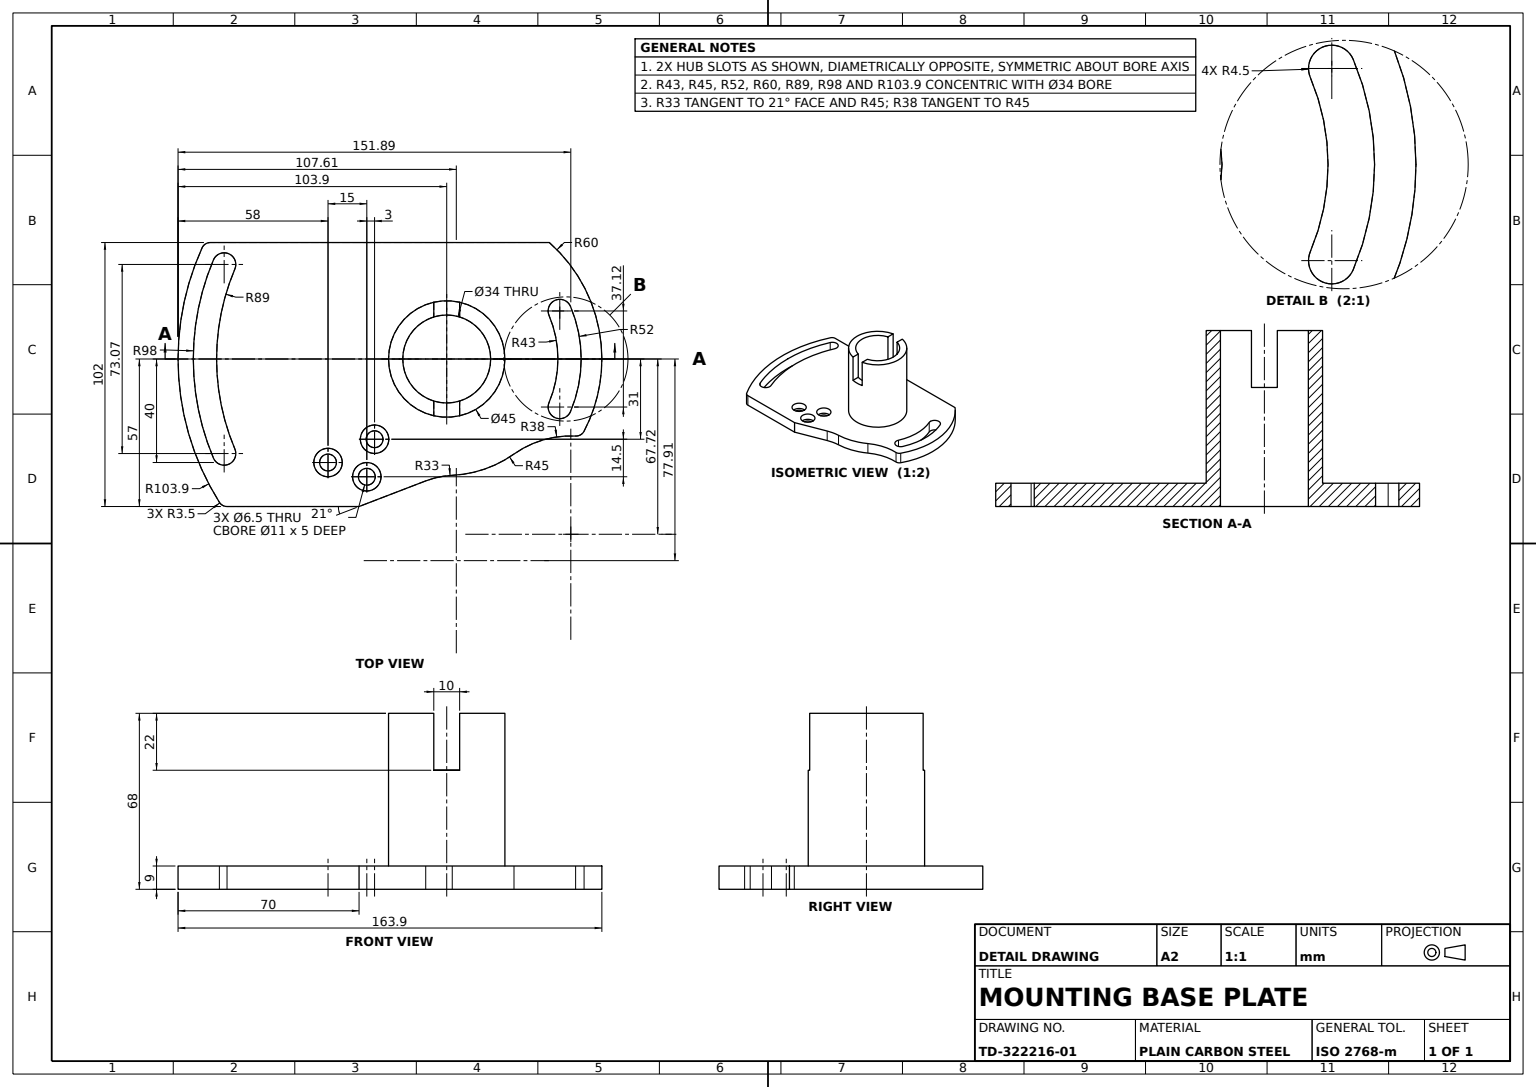
ISO-10303-21;
HEADER;
FILE_DESCRIPTION((''),'2;1');
FILE_NAME('','',(''),(''),'','','');
FILE_SCHEMA(('AUTOMOTIVE_DESIGN'));
ENDSEC;
DATA;
#1=APPLICATION_CONTEXT('');
#2=PRODUCT_CONTEXT('',#1,'mechanical');
#3=PRODUCT('','','',(#2));
#4=PRODUCT_DEFINITION_FORMATION('','',#3);
#5=PRODUCT_DEFINITION_CONTEXT('',#1,'design');
#6=PRODUCT_DEFINITION('','',#4,#5);
#7=PRODUCT_DEFINITION_SHAPE('','',#6);
#8=(LENGTH_UNIT()NAMED_UNIT(*)SI_UNIT(.MILLI.,.METRE.));
#9=(NAMED_UNIT(*)PLANE_ANGLE_UNIT()SI_UNIT($,.RADIAN.));
#10=(NAMED_UNIT(*)SI_UNIT($,.STERADIAN.)SOLID_ANGLE_UNIT());
#11=UNCERTAINTY_MEASURE_WITH_UNIT(LENGTH_MEASURE(1.E-05),#8,'distance_accuracy_value','');
#12=(GEOMETRIC_REPRESENTATION_CONTEXT(3)GLOBAL_UNCERTAINTY_ASSIGNED_CONTEXT((#11))GLOBAL_UNIT_ASSIGNED_CONTEXT((#8,#9,#10))REPRESENTATION_CONTEXT('',''));
#13=CARTESIAN_POINT('',(55.36504,0.,87.919977));
#14=VERTEX_POINT('',#13);
#15=CARTESIAN_POINT('',(57.,0.,84.958284));
#16=VERTEX_POINT('',#15);
#17=CARTESIAN_POINT('',(53.5,0.,84.958284));
#18=DIRECTION('',(0.,1.,0.));
#19=DIRECTION('',(0.,0.,-1.));
#20=AXIS2_PLACEMENT_3D('',#17,#18,#19);
#21=CIRCLE('',#20,3.5);
#22=EDGE_CURVE('',#14,#16,#21,.T.);
#23=ORIENTED_EDGE('',*,*,#22,.T.);
#24=CARTESIAN_POINT('',(57.,9.,84.958284));
#25=VERTEX_POINT('',#24);
#26=DIRECTION('',(0.,-1.,0.));
#27=VECTOR('',#26,1000.);
#28=LINE('',#24,#27);
#29=EDGE_CURVE('',#25,#16,#28,.T.);
#30=ORIENTED_EDGE('',*,*,#29,.F.);
#31=CARTESIAN_POINT('',(55.36504,9.,87.919977));
#32=VERTEX_POINT('',#31);
#33=CARTESIAN_POINT('',(53.5,9.,84.958284));
#34=AXIS2_PLACEMENT_3D('',#33,#18,#19);
#35=CIRCLE('',#34,3.5);
#36=EDGE_CURVE('',#32,#25,#35,.T.);
#37=ORIENTED_EDGE('',*,*,#36,.F.);
#38=LINE('',#31,#27);
#39=EDGE_CURVE('',#32,#14,#38,.T.);
#40=ORIENTED_EDGE('',*,*,#39,.T.);
#41=EDGE_LOOP('',(#23,#30,#37,#40));
#42=FACE_OUTER_BOUND('',#41,.T.);
#43=AXIS2_PLACEMENT_3D('',#33,#26,#19);
#44=CYLINDRICAL_SURFACE('',#43,3.5);
#45=ADVANCED_FACE('',(#42),#44,.T.);
#46=CARTESIAN_POINT('',(40.,4.,40.4));
#47=VERTEX_POINT('',#46);
#48=CARTESIAN_POINT('',(40.,4.,51.4));
#49=VERTEX_POINT('',#48);
#50=CARTESIAN_POINT('',(40.,4.,45.9));
#51=DIRECTION('',(0.,0.,1.));
#52=AXIS2_PLACEMENT_3D('',#50,#18,#51);
#53=CIRCLE('',#52,5.5);
#54=EDGE_CURVE('',#47,#49,#53,.T.);
#55=ORIENTED_EDGE('',*,*,#54,.F.);
#56=CARTESIAN_POINT('',(40.,9.,40.4));
#57=VERTEX_POINT('',#56);
#58=VECTOR('',#18,1000.);
#59=LINE('',#56,#58);
#60=EDGE_CURVE('',#47,#57,#59,.T.);
#61=ORIENTED_EDGE('',*,*,#60,.T.);
#62=CARTESIAN_POINT('',(40.,9.,51.4));
#63=VERTEX_POINT('',#62);
#64=CARTESIAN_POINT('',(40.,9.,45.9));
#65=AXIS2_PLACEMENT_3D('',#64,#18,#51);
#66=CIRCLE('',#65,5.5);
#67=EDGE_CURVE('',#57,#63,#66,.T.);
#68=ORIENTED_EDGE('',*,*,#67,.T.);
#69=LINE('',#62,#58);
#70=EDGE_CURVE('',#49,#63,#69,.T.);
#71=ORIENTED_EDGE('',*,*,#70,.F.);
#72=EDGE_LOOP('',(#55,#61,#68,#71));
#73=FACE_OUTER_BOUND('',#72,.T.);
#74=CYLINDRICAL_SURFACE('',#65,5.5);
#75=ADVANCED_FACE('',(#73),#74,.F.);
#76=CARTESIAN_POINT('',(21.937411,68.,-5.));
#77=VERTEX_POINT('',#76);
#78=CARTESIAN_POINT('',(0.,68.,-22.5));
#79=VERTEX_POINT('',#78);
#80=CARTESIAN_POINT('',(0.,68.,0.));
#81=AXIS2_PLACEMENT_3D('',#80,#18,#51);
#82=CIRCLE('',#81,22.5);
#83=EDGE_CURVE('',#77,#79,#82,.T.);
#84=ORIENTED_EDGE('',*,*,#83,.T.);
#85=CARTESIAN_POINT('',(-21.937411,68.,-5.));
#86=VERTEX_POINT('',#85);
#87=EDGE_CURVE('',#79,#86,#82,.T.);
#88=ORIENTED_EDGE('',*,*,#87,.T.);
#89=CARTESIAN_POINT('',(-16.248077,68.,-5.));
#90=VERTEX_POINT('',#89);
#91=CARTESIAN_POINT('',(-22.5,68.,-5.));
#92=DIRECTION('',(-1.,0.,0.));
#93=VECTOR('',#92,1000.);
#94=LINE('',#91,#93);
#95=EDGE_CURVE('',#90,#86,#94,.T.);
#96=ORIENTED_EDGE('',*,*,#95,.F.);
#97=CARTESIAN_POINT('',(0.,68.,-17.));
#98=VERTEX_POINT('',#97);
#99=CIRCLE('',#81,17.);
#100=EDGE_CURVE('',#98,#90,#99,.T.);
#101=ORIENTED_EDGE('',*,*,#100,.F.);
#102=CARTESIAN_POINT('',(16.248077,68.,-5.));
#103=VERTEX_POINT('',#102);
#104=EDGE_CURVE('',#103,#98,#99,.T.);
#105=ORIENTED_EDGE('',*,*,#104,.F.);
#106=EDGE_CURVE('',#77,#103,#94,.T.);
#107=ORIENTED_EDGE('',*,*,#106,.F.);
#108=EDGE_LOOP('',(#84,#88,#96,#101,#105,#107));
#109=FACE_OUTER_BOUND('',#108,.T.);
#110=PLANE('',#81);
#111=ADVANCED_FACE('',(#109),#110,.T.);
#112=CARTESIAN_POINT('',(18.559729,0.,-39.223981));
#113=VERTEX_POINT('',#112);
#114=CARTESIAN_POINT('',(18.559729,9.,-39.223981));
#115=VERTEX_POINT('',#114);
#116=CARTESIAN_POINT('',(18.559729,-0.001,-39.223981));
#117=LINE('',#116,#58);
#118=EDGE_CURVE('',#113,#115,#117,.T.);
#119=ORIENTED_EDGE('',*,*,#118,.F.);
#120=CARTESIAN_POINT('',(16.801439,0.,-39.581709));
#121=VERTEX_POINT('',#120);
#122=CARTESIAN_POINT('',(18.559729,0.,-43.723981));
#123=AXIS2_PLACEMENT_3D('',#122,#18,#19);
#124=CIRCLE('',#123,4.5);
#125=EDGE_CURVE('',#121,#113,#124,.T.);
#126=ORIENTED_EDGE('',*,*,#125,.F.);
#127=CARTESIAN_POINT('',(16.801439,9.,-39.581709));
#128=VERTEX_POINT('',#127);
#129=CARTESIAN_POINT('',(16.801439,-0.001,-39.581709));
#130=LINE('',#129,#58);
#131=EDGE_CURVE('',#121,#128,#130,.T.);
#132=ORIENTED_EDGE('',*,*,#131,.T.);
#133=CARTESIAN_POINT('',(18.559729,9.,-43.723981));
#134=AXIS2_PLACEMENT_3D('',#133,#18,#51);
#135=CIRCLE('',#134,4.5);
#136=EDGE_CURVE('',#128,#115,#135,.T.);
#137=ORIENTED_EDGE('',*,*,#136,.T.);
#138=EDGE_LOOP('',(#119,#126,#132,#137));
#139=FACE_OUTER_BOUND('',#138,.T.);
#140=CARTESIAN_POINT('',(18.559729,-0.001,-43.723981));
#141=AXIS2_PLACEMENT_3D('',#140,#18,#51);
#142=CYLINDRICAL_SURFACE('',#141,4.5);
#143=ADVANCED_FACE('',(#139),#142,.F.);
#144=CARTESIAN_POINT('',(47.103715,0.,8.119295));
#145=VERTEX_POINT('',#144);
#146=CARTESIAN_POINT('',(44.949155,0.,-2.138566));
#147=VERTEX_POINT('',#146);
#148=CARTESIAN_POINT('',(77.911869,0.,-3.706847));
#149=AXIS2_PLACEMENT_3D('',#148,#26,#19);
#150=CIRCLE('',#149,33.);
#151=EDGE_CURVE('',#145,#147,#150,.T.);
#152=ORIENTED_EDGE('',*,*,#151,.T.);
#153=CARTESIAN_POINT('',(44.949155,9.,-2.138566));
#154=VERTEX_POINT('',#153);
#155=LINE('',#153,#27);
#156=EDGE_CURVE('',#154,#147,#155,.T.);
#157=ORIENTED_EDGE('',*,*,#156,.F.);
#158=CARTESIAN_POINT('',(47.103715,9.,8.119295));
#159=VERTEX_POINT('',#158);
#160=CARTESIAN_POINT('',(77.911869,9.,-3.706847));
#161=AXIS2_PLACEMENT_3D('',#160,#26,#19);
#162=CIRCLE('',#161,33.);
#163=EDGE_CURVE('',#159,#154,#162,.T.);
#164=ORIENTED_EDGE('',*,*,#163,.F.);
#165=LINE('',#158,#27);
#166=EDGE_CURVE('',#159,#145,#165,.T.);
#167=ORIENTED_EDGE('',*,*,#166,.T.);
#168=EDGE_LOOP('',(#152,#157,#164,#167));
#169=FACE_OUTER_BOUND('',#168,.T.);
#170=CYLINDRICAL_SURFACE('',#161,33.);
#171=ADVANCED_FACE('',(#169),#170,.F.);
#172=CARTESIAN_POINT('',(-20.318019,0.,-47.866252));
#173=VERTEX_POINT('',#172);
#174=CARTESIAN_POINT('',(-20.318019,9.,-47.866252));
#175=VERTEX_POINT('',#174);
#176=CARTESIAN_POINT('',(-20.318019,-0.001,-47.866252));
#177=LINE('',#176,#58);
#178=EDGE_CURVE('',#173,#175,#177,.T.);
#179=ORIENTED_EDGE('',*,*,#178,.F.);
#180=CARTESIAN_POINT('',(20.318019,0.,-47.866252));
#181=VERTEX_POINT('',#180);
#182=CARTESIAN_POINT('',(0.,0.,0.));
#183=AXIS2_PLACEMENT_3D('',#182,#18,#19);
#184=CIRCLE('',#183,52.);
#185=EDGE_CURVE('',#181,#173,#184,.T.);
#186=ORIENTED_EDGE('',*,*,#185,.F.);
#187=CARTESIAN_POINT('',(20.318019,9.,-47.866252));
#188=VERTEX_POINT('',#187);
#189=CARTESIAN_POINT('',(20.318019,-0.001,-47.866252));
#190=LINE('',#189,#58);
#191=EDGE_CURVE('',#181,#188,#190,.T.);
#192=ORIENTED_EDGE('',*,*,#191,.T.);
#193=CARTESIAN_POINT('',(0.,9.,0.));
#194=AXIS2_PLACEMENT_3D('',#193,#18,#51);
#195=CIRCLE('',#194,52.);
#196=EDGE_CURVE('',#188,#175,#195,.T.);
#197=ORIENTED_EDGE('',*,*,#196,.T.);
#198=EDGE_LOOP('',(#179,#186,#192,#197));
#199=FACE_OUTER_BOUND('',#198,.T.);
#200=CARTESIAN_POINT('',(0.,-0.001,0.));
#201=AXIS2_PLACEMENT_3D('',#200,#18,#51);
#202=CYLINDRICAL_SURFACE('',#201,52.);
#203=ADVANCED_FACE('',(#199),#202,.F.);
#204=CARTESIAN_POINT('',(-16.248077,46.,5.));
#205=VERTEX_POINT('',#204);
#206=CARTESIAN_POINT('',(-16.248077,68.,5.));
#207=VERTEX_POINT('',#206);
#208=CARTESIAN_POINT('',(-16.248077,0.,5.));
#209=LINE('',#208,#58);
#210=EDGE_CURVE('',#205,#207,#209,.T.);
#211=ORIENTED_EDGE('',*,*,#210,.F.);
#212=CARTESIAN_POINT('',(-21.937411,46.,5.));
#213=VERTEX_POINT('',#212);
#214=CARTESIAN_POINT('',(-22.5,46.,5.));
#215=DIRECTION('',(1.,0.,0.));
#216=VECTOR('',#215,1000.);
#217=LINE('',#214,#216);
#218=EDGE_CURVE('',#213,#205,#217,.T.);
#219=ORIENTED_EDGE('',*,*,#218,.F.);
#220=CARTESIAN_POINT('',(-21.937411,68.,5.));
#221=VERTEX_POINT('',#220);
#222=LINE('',#220,#27);
#223=EDGE_CURVE('',#221,#213,#222,.T.);
#224=ORIENTED_EDGE('',*,*,#223,.F.);
#225=CARTESIAN_POINT('',(-22.5,68.,5.));
#226=LINE('',#225,#216);
#227=EDGE_CURVE('',#221,#207,#226,.T.);
#228=ORIENTED_EDGE('',*,*,#227,.T.);
#229=EDGE_LOOP('',(#211,#219,#224,#228));
#230=FACE_OUTER_BOUND('',#229,.T.);
#231=AXIS2_PLACEMENT_3D('',#214,#51,#215);
#232=PLANE('',#231);
#233=ADVANCED_FACE('',(#230),#232,.F.);
#234=ORIENTED_EDGE('',*,*,#218,.T.);
#235=CARTESIAN_POINT('',(-16.248077,46.,-5.));
#236=VERTEX_POINT('',#235);
#237=CARTESIAN_POINT('',(0.,46.,0.));
#238=AXIS2_PLACEMENT_3D('',#237,#18,#19);
#239=CIRCLE('',#238,17.);
#240=EDGE_CURVE('',#236,#205,#239,.T.);
#241=ORIENTED_EDGE('',*,*,#240,.F.);
#242=CARTESIAN_POINT('',(-21.937411,46.,-5.));
#243=VERTEX_POINT('',#242);
#244=CARTESIAN_POINT('',(-22.5,46.,-5.));
#245=LINE('',#244,#93);
#246=EDGE_CURVE('',#236,#243,#245,.T.);
#247=ORIENTED_EDGE('',*,*,#246,.T.);
#248=AXIS2_PLACEMENT_3D('',#237,#26,#19);
#249=CIRCLE('',#248,22.5);
#250=EDGE_CURVE('',#213,#243,#249,.T.);
#251=ORIENTED_EDGE('',*,*,#250,.F.);
#252=EDGE_LOOP('',(#234,#241,#247,#251));
#253=FACE_OUTER_BOUND('',#252,.T.);
#254=PLANE('',#248);
#255=ADVANCED_FACE('',(#253),#254,.F.);
#256=CARTESIAN_POINT('',(-38.291651,0.,90.209476));
#257=VERTEX_POINT('',#256);
#258=CARTESIAN_POINT('',(-38.291651,9.,90.209476));
#259=VERTEX_POINT('',#258);
#260=CARTESIAN_POINT('',(-38.291651,-0.001,90.209476));
#261=LINE('',#260,#58);
#262=EDGE_CURVE('',#257,#259,#261,.T.);
#263=ORIENTED_EDGE('',*,*,#262,.T.);
#264=CARTESIAN_POINT('',(0.,9.,98.));
#265=VERTEX_POINT('',#264);
#266=CIRCLE('',#194,98.);
#267=EDGE_CURVE('',#259,#265,#266,.T.);
#268=ORIENTED_EDGE('',*,*,#267,.T.);
#269=CARTESIAN_POINT('',(0.,0.,98.));
#270=VERTEX_POINT('',#269);
#271=CARTESIAN_POINT('',(0.,-0.001,98.));
#272=LINE('',#271,#58);
#273=EDGE_CURVE('',#270,#265,#272,.T.);
#274=ORIENTED_EDGE('',*,*,#273,.F.);
#275=CIRCLE('',#183,98.);
#276=EDGE_CURVE('',#257,#270,#275,.T.);
#277=ORIENTED_EDGE('',*,*,#276,.F.);
#278=EDGE_LOOP('',(#263,#268,#274,#277));
#279=FACE_OUTER_BOUND('',#278,.T.);
#280=CYLINDRICAL_SURFACE('',#201,98.);
#281=ADVANCED_FACE('',(#279),#280,.F.);
#282=CARTESIAN_POINT('',(21.937411,46.,5.));
#283=VERTEX_POINT('',#282);
#284=CARTESIAN_POINT('',(21.937411,68.,5.));
#285=VERTEX_POINT('',#284);
#286=LINE('',#284,#58);
#287=EDGE_CURVE('',#283,#285,#286,.T.);
#288=ORIENTED_EDGE('',*,*,#287,.F.);
#289=CARTESIAN_POINT('',(16.248077,46.,5.));
#290=VERTEX_POINT('',#289);
#291=EDGE_CURVE('',#290,#283,#217,.T.);
#292=ORIENTED_EDGE('',*,*,#291,.F.);
#293=CARTESIAN_POINT('',(16.248077,68.,5.));
#294=VERTEX_POINT('',#293);
#295=CARTESIAN_POINT('',(16.248077,0.,5.));
#296=LINE('',#295,#27);
#297=EDGE_CURVE('',#294,#290,#296,.T.);
#298=ORIENTED_EDGE('',*,*,#297,.F.);
#299=EDGE_CURVE('',#294,#285,#226,.T.);
#300=ORIENTED_EDGE('',*,*,#299,.T.);
#301=EDGE_LOOP('',(#288,#292,#298,#300));
#302=FACE_OUTER_BOUND('',#301,.T.);
#303=ADVANCED_FACE('',(#302),#232,.F.);
#304=CARTESIAN_POINT('',(45.5,4.,27.65));
#305=VERTEX_POINT('',#304);
#306=CARTESIAN_POINT('',(45.5,4.,34.15));
#307=VERTEX_POINT('',#306);
#308=CARTESIAN_POINT('',(45.5,4.,30.9));
#309=AXIS2_PLACEMENT_3D('',#308,#18,#51);
#310=CIRCLE('',#309,3.25);
#311=EDGE_CURVE('',#305,#307,#310,.T.);
#312=ORIENTED_EDGE('',*,*,#311,.F.);
#313=EDGE_CURVE('',#307,#305,#310,.T.);
#314=ORIENTED_EDGE('',*,*,#313,.F.);
#315=EDGE_LOOP('',(#312,#314));
#316=FACE_BOUND('',#315,.T.);
#317=CARTESIAN_POINT('',(45.5,4.,36.4));
#318=VERTEX_POINT('',#317);
#319=CARTESIAN_POINT('',(45.5,4.,25.4));
#320=VERTEX_POINT('',#319);
#321=CIRCLE('',#309,5.5);
#322=EDGE_CURVE('',#318,#320,#321,.T.);
#323=ORIENTED_EDGE('',*,*,#322,.T.);
#324=EDGE_CURVE('',#320,#318,#321,.T.);
#325=ORIENTED_EDGE('',*,*,#324,.T.);
#326=EDGE_LOOP('',(#323,#325));
#327=FACE_OUTER_BOUND('',#326,.T.);
#328=CARTESIAN_POINT('',(48.75,4.,30.9));
#329=AXIS2_PLACEMENT_3D('',#328,#26,#19);
#330=PLANE('',#329);
#331=ADVANCED_FACE('',(#316,#327),#330,.F.);
#332=ORIENTED_EDGE('',*,*,#246,.F.);
#333=CARTESIAN_POINT('',(-16.248077,0.,-5.));
#334=LINE('',#333,#27);
#335=EDGE_CURVE('',#90,#236,#334,.T.);
#336=ORIENTED_EDGE('',*,*,#335,.F.);
#337=ORIENTED_EDGE('',*,*,#95,.T.);
#338=LINE('',#85,#58);
#339=EDGE_CURVE('',#243,#86,#338,.T.);
#340=ORIENTED_EDGE('',*,*,#339,.F.);
#341=EDGE_LOOP('',(#332,#336,#337,#340));
#342=FACE_OUTER_BOUND('',#341,.T.);
#343=AXIS2_PLACEMENT_3D('',#244,#19,#92);
#344=PLANE('',#343);
#345=ADVANCED_FACE('',(#342),#344,.F.);
#346=ORIENTED_EDGE('',*,*,#313,.T.);
#347=CARTESIAN_POINT('',(45.5,0.,27.65));
#348=VERTEX_POINT('',#347);
#349=CARTESIAN_POINT('',(45.5,9.,27.65));
#350=LINE('',#349,#58);
#351=EDGE_CURVE('',#348,#305,#350,.T.);
#352=ORIENTED_EDGE('',*,*,#351,.F.);
#353=CARTESIAN_POINT('',(45.5,0.,34.15));
#354=VERTEX_POINT('',#353);
#355=CARTESIAN_POINT('',(45.5,0.,30.9));
#356=AXIS2_PLACEMENT_3D('',#355,#26,#19);
#357=CIRCLE('',#356,3.25);
#358=EDGE_CURVE('',#348,#354,#357,.T.);
#359=ORIENTED_EDGE('',*,*,#358,.T.);
#360=CARTESIAN_POINT('',(45.5,9.,34.15));
#361=LINE('',#360,#58);
#362=EDGE_CURVE('',#354,#307,#361,.T.);
#363=ORIENTED_EDGE('',*,*,#362,.T.);
#364=EDGE_LOOP('',(#346,#352,#359,#363));
#365=FACE_OUTER_BOUND('',#364,.T.);
#366=CARTESIAN_POINT('',(45.5,9.,30.9));
#367=AXIS2_PLACEMENT_3D('',#366,#18,#51);
#368=CYLINDRICAL_SURFACE('',#367,3.25);
#369=ADVANCED_FACE('',(#365),#368,.F.);
#370=CARTESIAN_POINT('',(0.,0.,-17.));
#371=VERTEX_POINT('',#370);
#372=LINE('',#370,#58);
#373=EDGE_CURVE('',#371,#98,#372,.T.);
#374=ORIENTED_EDGE('',*,*,#373,.T.);
#375=ORIENTED_EDGE('',*,*,#100,.T.);
#376=ORIENTED_EDGE('',*,*,#335,.T.);
#377=ORIENTED_EDGE('',*,*,#240,.T.);
#378=ORIENTED_EDGE('',*,*,#210,.T.);
#379=CARTESIAN_POINT('',(0.,68.,17.));
#380=VERTEX_POINT('',#379);
#381=EDGE_CURVE('',#207,#380,#99,.T.);
#382=ORIENTED_EDGE('',*,*,#381,.T.);
#383=CARTESIAN_POINT('',(0.,0.,17.));
#384=VERTEX_POINT('',#383);
#385=LINE('',#383,#58);
#386=EDGE_CURVE('',#384,#380,#385,.T.);
#387=ORIENTED_EDGE('',*,*,#386,.F.);
#388=AXIS2_PLACEMENT_3D('',#182,#18,#51);
#389=CIRCLE('',#388,17.);
#390=EDGE_CURVE('',#371,#384,#389,.T.);
#391=ORIENTED_EDGE('',*,*,#390,.F.);
#392=EDGE_LOOP('',(#374,#375,#376,#377,#378,#382,#387,#391));
#393=FACE_OUTER_BOUND('',#392,.T.);
#394=CYLINDRICAL_SURFACE('',#388,17.);
#395=ADVANCED_FACE('',(#393),#394,.F.);
#396=CARTESIAN_POINT('',(-18.559729,0.,-39.223981));
#397=VERTEX_POINT('',#396);
#398=CARTESIAN_POINT('',(-16.801439,0.,-39.581709));
#399=VERTEX_POINT('',#398);
#400=CARTESIAN_POINT('',(-18.559729,0.,-43.723981));
#401=AXIS2_PLACEMENT_3D('',#400,#18,#19);
#402=CIRCLE('',#401,4.5);
#403=EDGE_CURVE('',#397,#399,#402,.T.);
#404=ORIENTED_EDGE('',*,*,#403,.F.);
#405=CARTESIAN_POINT('',(-18.559729,9.,-39.223981));
#406=VERTEX_POINT('',#405);
#407=CARTESIAN_POINT('',(-18.559729,-0.001,-39.223981));
#408=LINE('',#407,#58);
#409=EDGE_CURVE('',#397,#406,#408,.T.);
#410=ORIENTED_EDGE('',*,*,#409,.T.);
#411=CARTESIAN_POINT('',(-16.801439,9.,-39.581709));
#412=VERTEX_POINT('',#411);
#413=CARTESIAN_POINT('',(-18.559729,9.,-43.723981));
#414=AXIS2_PLACEMENT_3D('',#413,#18,#51);
#415=CIRCLE('',#414,4.5);
#416=EDGE_CURVE('',#406,#412,#415,.T.);
#417=ORIENTED_EDGE('',*,*,#416,.T.);
#418=CARTESIAN_POINT('',(-16.801439,-0.001,-39.581709));
#419=LINE('',#418,#58);
#420=EDGE_CURVE('',#399,#412,#419,.T.);
#421=ORIENTED_EDGE('',*,*,#420,.F.);
#422=EDGE_LOOP('',(#404,#410,#417,#421));
#423=FACE_OUTER_BOUND('',#422,.T.);
#424=CARTESIAN_POINT('',(-18.559729,-0.001,-43.723981));
#425=AXIS2_PLACEMENT_3D('',#424,#18,#51);
#426=CYLINDRICAL_SURFACE('',#425,4.5);
#427=ADVANCED_FACE('',(#423),#426,.F.);
#428=EDGE_CURVE('',#173,#397,#402,.T.);
#429=ORIENTED_EDGE('',*,*,#428,.T.);
#430=ORIENTED_EDGE('',*,*,#403,.T.);
#431=AXIS2_PLACEMENT_3D('',#182,#26,#19);
#432=CIRCLE('',#431,43.);
#433=EDGE_CURVE('',#399,#121,#432,.T.);
#434=ORIENTED_EDGE('',*,*,#433,.T.);
#435=ORIENTED_EDGE('',*,*,#125,.T.);
#436=EDGE_CURVE('',#113,#181,#124,.T.);
#437=ORIENTED_EDGE('',*,*,#436,.T.);
#438=ORIENTED_EDGE('',*,*,#185,.T.);
#439=EDGE_LOOP('',(#429,#430,#434,#435,#437,#438));
#440=FACE_BOUND('',#439,.T.);
#441=CARTESIAN_POINT('',(40.,0.,42.65));
#442=VERTEX_POINT('',#441);
#443=CARTESIAN_POINT('',(40.,0.,49.15));
#444=VERTEX_POINT('',#443);
#445=CARTESIAN_POINT('',(40.,0.,45.9));
#446=AXIS2_PLACEMENT_3D('',#445,#26,#19);
#447=CIRCLE('',#446,3.25);
#448=EDGE_CURVE('',#442,#444,#447,.T.);
#449=ORIENTED_EDGE('',*,*,#448,.F.);
#450=EDGE_CURVE('',#444,#442,#447,.T.);
#451=ORIENTED_EDGE('',*,*,#450,.F.);
#452=EDGE_LOOP('',(#449,#451));
#453=FACE_BOUND('',#452,.T.);
#454=ORIENTED_EDGE('',*,*,#358,.F.);
#455=EDGE_CURVE('',#354,#348,#357,.T.);
#456=ORIENTED_EDGE('',*,*,#455,.F.);
#457=EDGE_LOOP('',(#454,#456));
#458=FACE_BOUND('',#457,.T.);
#459=ORIENTED_EDGE('',*,*,#390,.T.);
#460=EDGE_CURVE('',#384,#371,#389,.T.);
#461=ORIENTED_EDGE('',*,*,#460,.T.);
#462=EDGE_LOOP('',(#459,#461));
#463=FACE_BOUND('',#462,.T.);
#464=ORIENTED_EDGE('',*,*,#151,.F.);
#465=CARTESIAN_POINT('',(57.,0.,33.9));
#466=VERTEX_POINT('',#465);
#467=DIRECTION('',(-0.35836795,0.,-0.933580426));
#468=VECTOR('',#467,1000.);
#469=LINE('',#465,#468);
#470=EDGE_CURVE('',#466,#145,#469,.T.);
#471=ORIENTED_EDGE('',*,*,#470,.F.);
#472=VECTOR('',#19,1000.);
#473=LINE('',#15,#472);
#474=EDGE_CURVE('',#16,#466,#473,.T.);
#475=ORIENTED_EDGE('',*,*,#474,.F.);
#476=ORIENTED_EDGE('',*,*,#22,.F.);
#477=CARTESIAN_POINT('',(-42.946713,0.,94.608614));
#478=VERTEX_POINT('',#477);
#479=CIRCLE('',#388,103.9);
#480=EDGE_CURVE('',#478,#14,#479,.T.);
#481=ORIENTED_EDGE('',*,*,#480,.F.);
#482=CARTESIAN_POINT('',(-45.,0.,91.421606));
#483=VERTEX_POINT('',#482);
#484=CARTESIAN_POINT('',(-41.5,0.,91.421606));
#485=AXIS2_PLACEMENT_3D('',#484,#18,#51);
#486=CIRCLE('',#485,3.5);
#487=EDGE_CURVE('',#483,#478,#486,.T.);
#488=ORIENTED_EDGE('',*,*,#487,.F.);
#489=CARTESIAN_POINT('',(-45.,0.,-39.685663));
#490=VERTEX_POINT('',#489);
#491=VECTOR('',#51,1000.);
#492=LINE('',#489,#491);
#493=EDGE_CURVE('',#490,#483,#492,.T.);
#494=ORIENTED_EDGE('',*,*,#493,.F.);
#495=CARTESIAN_POINT('',(0.,0.,-59.999599));
#496=VERTEX_POINT('',#495);
#497=CIRCLE('',#183,59.999599);
#498=EDGE_CURVE('',#496,#490,#497,.T.);
#499=ORIENTED_EDGE('',*,*,#498,.F.);
#500=CARTESIAN_POINT('',(27.897091,0.,-53.119715));
#501=VERTEX_POINT('',#500);
#502=EDGE_CURVE('',#501,#496,#497,.T.);
#503=ORIENTED_EDGE('',*,*,#502,.F.);
#504=CARTESIAN_POINT('',(29.765554,0.,-49.849718));
#505=VERTEX_POINT('',#504);
#506=CARTESIAN_POINT('',(26.26975,0.,-50.021045));
#507=AXIS2_PLACEMENT_3D('',#506,#18,#51);
#508=CIRCLE('',#507,3.5);
#509=EDGE_CURVE('',#505,#501,#508,.T.);
#510=ORIENTED_EDGE('',*,*,#509,.F.);
#511=CARTESIAN_POINT('',(36.715663,0.,-26.018457));
#512=VERTEX_POINT('',#511);
#513=CARTESIAN_POINT('',(67.72,0.,-47.989599));
#514=AXIS2_PLACEMENT_3D('',#513,#26,#51);
#515=CIRCLE('',#514,38.);
#516=EDGE_CURVE('',#512,#505,#515,.T.);
#517=ORIENTED_EDGE('',*,*,#516,.F.);
#518=CIRCLE('',#388,45.);
#519=EDGE_CURVE('',#147,#512,#518,.T.);
#520=ORIENTED_EDGE('',*,*,#519,.F.);
#521=EDGE_LOOP('',(#464,#471,#475,#476,#481,#488,#494,#499,#503,#510,#517,#520));
#522=FACE_OUTER_BOUND('',#521,.T.);
#523=CARTESIAN_POINT('',(31.,0.,24.65));
#524=VERTEX_POINT('',#523);
#525=CARTESIAN_POINT('',(31.,0.,31.15));
#526=VERTEX_POINT('',#525);
#527=CARTESIAN_POINT('',(31.,0.,27.9));
#528=AXIS2_PLACEMENT_3D('',#527,#26,#19);
#529=CIRCLE('',#528,3.25);
#530=EDGE_CURVE('',#524,#526,#529,.T.);
#531=ORIENTED_EDGE('',*,*,#530,.F.);
#532=EDGE_CURVE('',#526,#524,#529,.T.);
#533=ORIENTED_EDGE('',*,*,#532,.F.);
#534=EDGE_LOOP('',(#531,#533));
#535=FACE_BOUND('',#534,.T.);
#536=CARTESIAN_POINT('',(0.,0.,89.));
#537=VERTEX_POINT('',#536);
#538=CARTESIAN_POINT('',(-34.77507,0.,81.924932));
#539=VERTEX_POINT('',#538);
#540=CIRCLE('',#431,89.);
#541=EDGE_CURVE('',#537,#539,#540,.T.);
#542=ORIENTED_EDGE('',*,*,#541,.T.);
#543=CARTESIAN_POINT('',(-36.533361,0.,86.067204));
#544=AXIS2_PLACEMENT_3D('',#543,#18,#19);
#545=CIRCLE('',#544,4.5);
#546=EDGE_CURVE('',#539,#257,#545,.T.);
#547=ORIENTED_EDGE('',*,*,#546,.T.);
#548=ORIENTED_EDGE('',*,*,#276,.T.);
#549=CARTESIAN_POINT('',(38.291651,0.,90.209476));
#550=VERTEX_POINT('',#549);
#551=EDGE_CURVE('',#270,#550,#275,.T.);
#552=ORIENTED_EDGE('',*,*,#551,.T.);
#553=CARTESIAN_POINT('',(34.77507,0.,81.924932));
#554=VERTEX_POINT('',#553);
#555=CARTESIAN_POINT('',(36.533361,0.,86.067204));
#556=AXIS2_PLACEMENT_3D('',#555,#18,#19);
#557=CIRCLE('',#556,4.5);
#558=EDGE_CURVE('',#550,#554,#557,.T.);
#559=ORIENTED_EDGE('',*,*,#558,.T.);
#560=EDGE_CURVE('',#554,#537,#540,.T.);
#561=ORIENTED_EDGE('',*,*,#560,.T.);
#562=EDGE_LOOP('',(#542,#547,#548,#552,#559,#561));
#563=FACE_BOUND('',#562,.T.);
#564=AXIS2_PLACEMENT_3D('',#17,#26,#19);
#565=PLANE('',#564);
#566=ADVANCED_FACE('',(#440,#453,#458,#463,#522,#535,#563),#565,.T.);
#567=CARTESIAN_POINT('',(40.,4.,49.15));
#568=VERTEX_POINT('',#567);
#569=CARTESIAN_POINT('',(40.,4.,42.65));
#570=VERTEX_POINT('',#569);
#571=CIRCLE('',#52,3.25);
#572=EDGE_CURVE('',#568,#570,#571,.T.);
#573=ORIENTED_EDGE('',*,*,#572,.F.);
#574=EDGE_CURVE('',#570,#568,#571,.T.);
#575=ORIENTED_EDGE('',*,*,#574,.F.);
#576=EDGE_LOOP('',(#573,#575));
#577=FACE_BOUND('',#576,.T.);
#578=EDGE_CURVE('',#49,#47,#53,.T.);
#579=ORIENTED_EDGE('',*,*,#578,.T.);
#580=ORIENTED_EDGE('',*,*,#54,.T.);
#581=EDGE_LOOP('',(#579,#580));
#582=FACE_OUTER_BOUND('',#581,.T.);
#583=CARTESIAN_POINT('',(43.25,4.,45.9));
#584=AXIS2_PLACEMENT_3D('',#583,#26,#19);
#585=PLANE('',#584);
#586=ADVANCED_FACE('',(#577,#582),#585,.F.);
#587=CARTESIAN_POINT('',(-45.,9.,91.421606));
#588=VERTEX_POINT('',#587);
#589=CARTESIAN_POINT('',(-42.946713,9.,94.608614));
#590=VERTEX_POINT('',#589);
#591=CARTESIAN_POINT('',(-41.5,9.,91.421606));
#592=AXIS2_PLACEMENT_3D('',#591,#18,#51);
#593=CIRCLE('',#592,3.5);
#594=EDGE_CURVE('',#588,#590,#593,.T.);
#595=ORIENTED_EDGE('',*,*,#594,.F.);
#596=LINE('',#587,#27);
#597=EDGE_CURVE('',#588,#483,#596,.T.);
#598=ORIENTED_EDGE('',*,*,#597,.T.);
#599=ORIENTED_EDGE('',*,*,#487,.T.);
#600=LINE('',#589,#27);
#601=EDGE_CURVE('',#590,#478,#600,.T.);
#602=ORIENTED_EDGE('',*,*,#601,.F.);
#603=EDGE_LOOP('',(#595,#598,#599,#602));
#604=FACE_OUTER_BOUND('',#603,.T.);
#605=AXIS2_PLACEMENT_3D('',#591,#26,#19);
#606=CYLINDRICAL_SURFACE('',#605,3.5);
#607=ADVANCED_FACE('',(#604),#606,.T.);
#608=CARTESIAN_POINT('',(-34.77507,9.,81.924932));
#609=VERTEX_POINT('',#608);
#610=CARTESIAN_POINT('',(-34.77507,-0.001,81.924932));
#611=LINE('',#610,#58);
#612=EDGE_CURVE('',#539,#609,#611,.T.);
#613=ORIENTED_EDGE('',*,*,#612,.F.);
#614=ORIENTED_EDGE('',*,*,#541,.F.);
#615=CARTESIAN_POINT('',(0.,9.,89.));
#616=VERTEX_POINT('',#615);
#617=CARTESIAN_POINT('',(0.,-0.001,89.));
#618=LINE('',#617,#58);
#619=EDGE_CURVE('',#537,#616,#618,.T.);
#620=ORIENTED_EDGE('',*,*,#619,.T.);
#621=AXIS2_PLACEMENT_3D('',#193,#26,#51);
#622=CIRCLE('',#621,89.);
#623=EDGE_CURVE('',#616,#609,#622,.T.);
#624=ORIENTED_EDGE('',*,*,#623,.T.);
#625=EDGE_LOOP('',(#613,#614,#620,#624));
#626=FACE_OUTER_BOUND('',#625,.T.);
#627=CYLINDRICAL_SURFACE('',#201,89.);
#628=ADVANCED_FACE('',(#626),#627,.T.);
#629=ORIENTED_EDGE('',*,*,#299,.F.);
#630=EDGE_CURVE('',#380,#294,#99,.T.);
#631=ORIENTED_EDGE('',*,*,#630,.F.);
#632=ORIENTED_EDGE('',*,*,#381,.F.);
#633=ORIENTED_EDGE('',*,*,#227,.F.);
#634=CARTESIAN_POINT('',(0.,68.,22.5));
#635=VERTEX_POINT('',#634);
#636=EDGE_CURVE('',#221,#635,#82,.T.);
#637=ORIENTED_EDGE('',*,*,#636,.T.);
#638=EDGE_CURVE('',#635,#285,#82,.T.);
#639=ORIENTED_EDGE('',*,*,#638,.T.);
#640=EDGE_LOOP('',(#629,#631,#632,#633,#637,#639));
#641=FACE_OUTER_BOUND('',#640,.T.);
#642=ADVANCED_FACE('',(#641),#110,.T.);
#643=CARTESIAN_POINT('',(-45.,9.,-39.685663));
#644=VERTEX_POINT('',#643);
#645=LINE('',#643,#491);
#646=EDGE_CURVE('',#644,#588,#645,.T.);
#647=ORIENTED_EDGE('',*,*,#646,.F.);
#648=LINE('',#643,#27);
#649=EDGE_CURVE('',#644,#490,#648,.T.);
#650=ORIENTED_EDGE('',*,*,#649,.T.);
#651=ORIENTED_EDGE('',*,*,#493,.T.);
#652=ORIENTED_EDGE('',*,*,#597,.F.);
#653=EDGE_LOOP('',(#647,#650,#651,#652));
#654=FACE_OUTER_BOUND('',#653,.T.);
#655=AXIS2_PLACEMENT_3D('',#643,#215,#19);
#656=PLANE('',#655);
#657=ADVANCED_FACE('',(#654),#656,.F.);
#658=CARTESIAN_POINT('',(31.,4.,31.15));
#659=VERTEX_POINT('',#658);
#660=CARTESIAN_POINT('',(31.,4.,24.65));
#661=VERTEX_POINT('',#660);
#662=CARTESIAN_POINT('',(31.,4.,27.9));
#663=AXIS2_PLACEMENT_3D('',#662,#18,#51);
#664=CIRCLE('',#663,3.25);
#665=EDGE_CURVE('',#659,#661,#664,.T.);
#666=ORIENTED_EDGE('',*,*,#665,.F.);
#667=EDGE_CURVE('',#661,#659,#664,.T.);
#668=ORIENTED_EDGE('',*,*,#667,.F.);
#669=EDGE_LOOP('',(#666,#668));
#670=FACE_BOUND('',#669,.T.);
#671=CARTESIAN_POINT('',(31.,4.,22.4));
#672=VERTEX_POINT('',#671);
#673=CARTESIAN_POINT('',(31.,4.,33.4));
#674=VERTEX_POINT('',#673);
#675=CIRCLE('',#663,5.5);
#676=EDGE_CURVE('',#672,#674,#675,.T.);
#677=ORIENTED_EDGE('',*,*,#676,.T.);
#678=EDGE_CURVE('',#674,#672,#675,.T.);
#679=ORIENTED_EDGE('',*,*,#678,.T.);
#680=EDGE_LOOP('',(#677,#679));
#681=FACE_OUTER_BOUND('',#680,.T.);
#682=CARTESIAN_POINT('',(34.25,4.,27.9));
#683=AXIS2_PLACEMENT_3D('',#682,#26,#19);
#684=PLANE('',#683);
#685=ADVANCED_FACE('',(#670,#681),#684,.F.);
#686=ORIENTED_EDGE('',*,*,#636,.F.);
#687=ORIENTED_EDGE('',*,*,#223,.T.);
#688=ORIENTED_EDGE('',*,*,#250,.T.);
#689=ORIENTED_EDGE('',*,*,#339,.T.);
#690=ORIENTED_EDGE('',*,*,#87,.F.);
#691=CARTESIAN_POINT('',(0.,9.,-22.5));
#692=VERTEX_POINT('',#691);
#693=LINE('',#78,#27);
#694=EDGE_CURVE('',#79,#692,#693,.T.);
#695=ORIENTED_EDGE('',*,*,#694,.T.);
#696=CARTESIAN_POINT('',(0.,9.,22.5));
#697=VERTEX_POINT('',#696);
#698=AXIS2_PLACEMENT_3D('',#193,#18,#19);
#699=CIRCLE('',#698,22.5);
#700=EDGE_CURVE('',#692,#697,#699,.T.);
#701=ORIENTED_EDGE('',*,*,#700,.T.);
#702=LINE('',#634,#27);
#703=EDGE_CURVE('',#635,#697,#702,.T.);
#704=ORIENTED_EDGE('',*,*,#703,.F.);
#705=EDGE_LOOP('',(#686,#687,#688,#689,#690,#695,#701,#704));
#706=FACE_OUTER_BOUND('',#705,.T.);
#707=AXIS2_PLACEMENT_3D('',#80,#26,#19);
#708=CYLINDRICAL_SURFACE('',#707,22.5);
#709=ADVANCED_FACE('',(#706),#708,.T.);
#710=CARTESIAN_POINT('',(31.,9.,31.15));
#711=LINE('',#710,#58);
#712=EDGE_CURVE('',#526,#659,#711,.T.);
#713=ORIENTED_EDGE('',*,*,#712,.F.);
#714=ORIENTED_EDGE('',*,*,#532,.T.);
#715=CARTESIAN_POINT('',(31.,9.,24.65));
#716=LINE('',#715,#58);
#717=EDGE_CURVE('',#524,#661,#716,.T.);
#718=ORIENTED_EDGE('',*,*,#717,.T.);
#719=ORIENTED_EDGE('',*,*,#667,.T.);
#720=EDGE_LOOP('',(#713,#714,#718,#719));
#721=FACE_OUTER_BOUND('',#720,.T.);
#722=CARTESIAN_POINT('',(31.,9.,27.9));
#723=AXIS2_PLACEMENT_3D('',#722,#18,#51);
#724=CYLINDRICAL_SURFACE('',#723,3.25);
#725=ADVANCED_FACE('',(#721),#724,.F.);
#726=ORIENTED_EDGE('',*,*,#619,.F.);
#727=ORIENTED_EDGE('',*,*,#560,.F.);
#728=CARTESIAN_POINT('',(34.77507,9.,81.924932));
#729=VERTEX_POINT('',#728);
#730=CARTESIAN_POINT('',(34.77507,-0.001,81.924932));
#731=LINE('',#730,#58);
#732=EDGE_CURVE('',#554,#729,#731,.T.);
#733=ORIENTED_EDGE('',*,*,#732,.T.);
#734=EDGE_CURVE('',#729,#616,#622,.T.);
#735=ORIENTED_EDGE('',*,*,#734,.T.);
#736=EDGE_LOOP('',(#726,#727,#733,#735));
#737=FACE_OUTER_BOUND('',#736,.T.);
#738=ADVANCED_FACE('',(#737),#627,.T.);
#739=CARTESIAN_POINT('',(45.5,9.,36.4));
#740=VERTEX_POINT('',#739);
#741=CARTESIAN_POINT('',(45.5,9.,25.4));
#742=VERTEX_POINT('',#741);
#743=CIRCLE('',#367,5.5);
#744=EDGE_CURVE('',#740,#742,#743,.T.);
#745=ORIENTED_EDGE('',*,*,#744,.T.);
#746=LINE('',#741,#58);
#747=EDGE_CURVE('',#320,#742,#746,.T.);
#748=ORIENTED_EDGE('',*,*,#747,.F.);
#749=ORIENTED_EDGE('',*,*,#322,.F.);
#750=LINE('',#739,#58);
#751=EDGE_CURVE('',#318,#740,#750,.T.);
#752=ORIENTED_EDGE('',*,*,#751,.T.);
#753=EDGE_LOOP('',(#745,#748,#749,#752));
#754=FACE_OUTER_BOUND('',#753,.T.);
#755=CYLINDRICAL_SURFACE('',#367,5.5);
#756=ADVANCED_FACE('',(#754),#755,.F.);
#757=ORIENTED_EDGE('',*,*,#703,.T.);
#758=EDGE_CURVE('',#697,#692,#699,.T.);
#759=ORIENTED_EDGE('',*,*,#758,.T.);
#760=ORIENTED_EDGE('',*,*,#694,.F.);
#761=ORIENTED_EDGE('',*,*,#83,.F.);
#762=CARTESIAN_POINT('',(21.937411,46.,-5.));
#763=VERTEX_POINT('',#762);
#764=LINE('',#76,#27);
#765=EDGE_CURVE('',#77,#763,#764,.T.);
#766=ORIENTED_EDGE('',*,*,#765,.T.);
#767=EDGE_CURVE('',#763,#283,#249,.T.);
#768=ORIENTED_EDGE('',*,*,#767,.T.);
#769=ORIENTED_EDGE('',*,*,#287,.T.);
#770=ORIENTED_EDGE('',*,*,#638,.F.);
#771=EDGE_LOOP('',(#757,#759,#760,#761,#766,#768,#769,#770));
#772=FACE_OUTER_BOUND('',#771,.T.);
#773=ADVANCED_FACE('',(#772),#708,.T.);
#774=ORIENTED_EDGE('',*,*,#362,.F.);
#775=ORIENTED_EDGE('',*,*,#455,.T.);
#776=ORIENTED_EDGE('',*,*,#351,.T.);
#777=ORIENTED_EDGE('',*,*,#311,.T.);
#778=EDGE_LOOP('',(#774,#775,#776,#777));
#779=FACE_OUTER_BOUND('',#778,.T.);
#780=ADVANCED_FACE('',(#779),#368,.F.);
#781=ORIENTED_EDGE('',*,*,#118,.T.);
#782=EDGE_CURVE('',#115,#188,#135,.T.);
#783=ORIENTED_EDGE('',*,*,#782,.T.);
#784=ORIENTED_EDGE('',*,*,#191,.F.);
#785=ORIENTED_EDGE('',*,*,#436,.F.);
#786=EDGE_LOOP('',(#781,#783,#784,#785));
#787=FACE_OUTER_BOUND('',#786,.T.);
#788=ADVANCED_FACE('',(#787),#142,.F.);
#789=ORIENTED_EDGE('',*,*,#502,.T.);
#790=CARTESIAN_POINT('',(0.,9.,-59.999599));
#791=VERTEX_POINT('',#790);
#792=LINE('',#790,#27);
#793=EDGE_CURVE('',#791,#496,#792,.T.);
#794=ORIENTED_EDGE('',*,*,#793,.F.);
#795=CARTESIAN_POINT('',(27.897091,9.,-53.119715));
#796=VERTEX_POINT('',#795);
#797=CIRCLE('',#698,59.999599);
#798=EDGE_CURVE('',#796,#791,#797,.T.);
#799=ORIENTED_EDGE('',*,*,#798,.F.);
#800=LINE('',#795,#27);
#801=EDGE_CURVE('',#796,#501,#800,.T.);
#802=ORIENTED_EDGE('',*,*,#801,.T.);
#803=EDGE_LOOP('',(#789,#794,#799,#802));
#804=FACE_OUTER_BOUND('',#803,.T.);
#805=AXIS2_PLACEMENT_3D('',#193,#26,#19);
#806=CYLINDRICAL_SURFACE('',#805,59.999599);
#807=ADVANCED_FACE('',(#804),#806,.T.);
#808=ORIENTED_EDGE('',*,*,#29,.T.);
#809=ORIENTED_EDGE('',*,*,#474,.T.);
#810=CARTESIAN_POINT('',(57.,9.,33.9));
#811=VERTEX_POINT('',#810);
#812=LINE('',#810,#27);
#813=EDGE_CURVE('',#811,#466,#812,.T.);
#814=ORIENTED_EDGE('',*,*,#813,.F.);
#815=LINE('',#24,#472);
#816=EDGE_CURVE('',#25,#811,#815,.T.);
#817=ORIENTED_EDGE('',*,*,#816,.F.);
#818=EDGE_LOOP('',(#808,#809,#814,#817));
#819=FACE_OUTER_BOUND('',#818,.T.);
#820=AXIS2_PLACEMENT_3D('',#24,#92,#51);
#821=PLANE('',#820);
#822=ADVANCED_FACE('',(#819),#821,.F.);
#823=ORIENTED_EDGE('',*,*,#649,.F.);
#824=EDGE_CURVE('',#791,#644,#797,.T.);
#825=ORIENTED_EDGE('',*,*,#824,.F.);
#826=ORIENTED_EDGE('',*,*,#793,.T.);
#827=ORIENTED_EDGE('',*,*,#498,.T.);
#828=EDGE_LOOP('',(#823,#825,#826,#827));
#829=FACE_OUTER_BOUND('',#828,.T.);
#830=ADVANCED_FACE('',(#829),#806,.T.);
#831=CARTESIAN_POINT('',(31.,9.,22.4));
#832=VERTEX_POINT('',#831);
#833=LINE('',#831,#58);
#834=EDGE_CURVE('',#672,#832,#833,.T.);
#835=ORIENTED_EDGE('',*,*,#834,.F.);
#836=ORIENTED_EDGE('',*,*,#678,.F.);
#837=CARTESIAN_POINT('',(31.,9.,33.4));
#838=VERTEX_POINT('',#837);
#839=LINE('',#837,#58);
#840=EDGE_CURVE('',#674,#838,#839,.T.);
#841=ORIENTED_EDGE('',*,*,#840,.T.);
#842=CIRCLE('',#723,5.5);
#843=EDGE_CURVE('',#838,#832,#842,.T.);
#844=ORIENTED_EDGE('',*,*,#843,.T.);
#845=EDGE_LOOP('',(#835,#836,#841,#844));
#846=FACE_OUTER_BOUND('',#845,.T.);
#847=CYLINDRICAL_SURFACE('',#723,5.5);
#848=ADVANCED_FACE('',(#846),#847,.F.);
#849=ORIENTED_EDGE('',*,*,#767,.F.);
#850=CARTESIAN_POINT('',(16.248077,46.,-5.));
#851=VERTEX_POINT('',#850);
#852=EDGE_CURVE('',#763,#851,#245,.T.);
#853=ORIENTED_EDGE('',*,*,#852,.T.);
#854=EDGE_CURVE('',#290,#851,#239,.T.);
#855=ORIENTED_EDGE('',*,*,#854,.F.);
#856=ORIENTED_EDGE('',*,*,#291,.T.);
#857=EDGE_LOOP('',(#849,#853,#855,#856));
#858=FACE_OUTER_BOUND('',#857,.T.);
#859=ADVANCED_FACE('',(#858),#254,.F.);
#860=CARTESIAN_POINT('',(36.715663,9.,-26.018457));
#861=VERTEX_POINT('',#860);
#862=LINE('',#860,#27);
#863=EDGE_CURVE('',#861,#512,#862,.T.);
#864=ORIENTED_EDGE('',*,*,#863,.T.);
#865=ORIENTED_EDGE('',*,*,#516,.T.);
#866=CARTESIAN_POINT('',(29.765554,9.,-49.849718));
#867=VERTEX_POINT('',#866);
#868=LINE('',#866,#27);
#869=EDGE_CURVE('',#867,#505,#868,.T.);
#870=ORIENTED_EDGE('',*,*,#869,.F.);
#871=CARTESIAN_POINT('',(67.72,9.,-47.989599));
#872=AXIS2_PLACEMENT_3D('',#871,#26,#51);
#873=CIRCLE('',#872,38.);
#874=EDGE_CURVE('',#861,#867,#873,.T.);
#875=ORIENTED_EDGE('',*,*,#874,.F.);
#876=EDGE_LOOP('',(#864,#865,#870,#875));
#877=FACE_OUTER_BOUND('',#876,.T.);
#878=AXIS2_PLACEMENT_3D('',#871,#26,#19);
#879=CYLINDRICAL_SURFACE('',#878,38.);
#880=ADVANCED_FACE('',(#877),#879,.F.);
#881=ORIENTED_EDGE('',*,*,#732,.F.);
#882=ORIENTED_EDGE('',*,*,#558,.F.);
#883=CARTESIAN_POINT('',(38.291651,9.,90.209476));
#884=VERTEX_POINT('',#883);
#885=CARTESIAN_POINT('',(38.291651,-0.001,90.209476));
#886=LINE('',#885,#58);
#887=EDGE_CURVE('',#550,#884,#886,.T.);
#888=ORIENTED_EDGE('',*,*,#887,.T.);
#889=CARTESIAN_POINT('',(36.533361,9.,86.067204));
#890=AXIS2_PLACEMENT_3D('',#889,#18,#51);
#891=CIRCLE('',#890,4.5);
#892=EDGE_CURVE('',#884,#729,#891,.T.);
#893=ORIENTED_EDGE('',*,*,#892,.T.);
#894=EDGE_LOOP('',(#881,#882,#888,#893));
#895=FACE_OUTER_BOUND('',#894,.T.);
#896=CARTESIAN_POINT('',(36.533361,-0.001,86.067204));
#897=AXIS2_PLACEMENT_3D('',#896,#18,#51);
#898=CYLINDRICAL_SURFACE('',#897,4.5);
#899=ADVANCED_FACE('',(#895),#898,.F.);
#900=ORIENTED_EDGE('',*,*,#546,.F.);
#901=ORIENTED_EDGE('',*,*,#612,.T.);
#902=CARTESIAN_POINT('',(-36.533361,9.,86.067204));
#903=AXIS2_PLACEMENT_3D('',#902,#18,#51);
#904=CIRCLE('',#903,4.5);
#905=EDGE_CURVE('',#609,#259,#904,.T.);
#906=ORIENTED_EDGE('',*,*,#905,.T.);
#907=ORIENTED_EDGE('',*,*,#262,.F.);
#908=EDGE_LOOP('',(#900,#901,#906,#907));
#909=FACE_OUTER_BOUND('',#908,.T.);
#910=CARTESIAN_POINT('',(-36.533361,-0.001,86.067204));
#911=AXIS2_PLACEMENT_3D('',#910,#18,#51);
#912=CYLINDRICAL_SURFACE('',#911,4.5);
#913=ADVANCED_FACE('',(#909),#912,.F.);
#914=ORIENTED_EDGE('',*,*,#480,.T.);
#915=ORIENTED_EDGE('',*,*,#39,.F.);
#916=CIRCLE('',#194,103.9);
#917=EDGE_CURVE('',#590,#32,#916,.T.);
#918=ORIENTED_EDGE('',*,*,#917,.F.);
#919=ORIENTED_EDGE('',*,*,#601,.T.);
#920=EDGE_LOOP('',(#914,#915,#918,#919));
#921=FACE_OUTER_BOUND('',#920,.T.);
#922=CYLINDRICAL_SURFACE('',#805,103.9);
#923=ADVANCED_FACE('',(#921),#922,.T.);
#924=ORIENTED_EDGE('',*,*,#386,.T.);
#925=ORIENTED_EDGE('',*,*,#630,.T.);
#926=ORIENTED_EDGE('',*,*,#297,.T.);
#927=ORIENTED_EDGE('',*,*,#854,.T.);
#928=CARTESIAN_POINT('',(16.248077,0.,-5.));
#929=LINE('',#928,#58);
#930=EDGE_CURVE('',#851,#103,#929,.T.);
#931=ORIENTED_EDGE('',*,*,#930,.T.);
#932=ORIENTED_EDGE('',*,*,#104,.T.);
#933=ORIENTED_EDGE('',*,*,#373,.F.);
#934=ORIENTED_EDGE('',*,*,#460,.F.);
#935=EDGE_LOOP('',(#924,#925,#926,#927,#931,#932,#933,#934));
#936=FACE_OUTER_BOUND('',#935,.T.);
#937=ADVANCED_FACE('',(#936),#394,.F.);
#938=ORIENTED_EDGE('',*,*,#178,.T.);
#939=EDGE_CURVE('',#175,#406,#415,.T.);
#940=ORIENTED_EDGE('',*,*,#939,.T.);
#941=ORIENTED_EDGE('',*,*,#409,.F.);
#942=ORIENTED_EDGE('',*,*,#428,.F.);
#943=EDGE_LOOP('',(#938,#940,#941,#942));
#944=FACE_OUTER_BOUND('',#943,.T.);
#945=ADVANCED_FACE('',(#944),#426,.F.);
#946=EDGE_CURVE('',#832,#838,#842,.T.);
#947=ORIENTED_EDGE('',*,*,#946,.T.);
#948=ORIENTED_EDGE('',*,*,#840,.F.);
#949=ORIENTED_EDGE('',*,*,#676,.F.);
#950=ORIENTED_EDGE('',*,*,#834,.T.);
#951=EDGE_LOOP('',(#947,#948,#949,#950));
#952=FACE_OUTER_BOUND('',#951,.T.);
#953=ADVANCED_FACE('',(#952),#847,.F.);
#954=ORIENTED_EDGE('',*,*,#324,.F.);
#955=ORIENTED_EDGE('',*,*,#747,.T.);
#956=EDGE_CURVE('',#742,#740,#743,.T.);
#957=ORIENTED_EDGE('',*,*,#956,.T.);
#958=ORIENTED_EDGE('',*,*,#751,.F.);
#959=EDGE_LOOP('',(#954,#955,#957,#958));
#960=FACE_OUTER_BOUND('',#959,.T.);
#961=ADVANCED_FACE('',(#960),#755,.F.);
#962=ORIENTED_EDGE('',*,*,#136,.F.);
#963=CIRCLE('',#621,43.);
#964=EDGE_CURVE('',#412,#128,#963,.T.);
#965=ORIENTED_EDGE('',*,*,#964,.F.);
#966=ORIENTED_EDGE('',*,*,#416,.F.);
#967=ORIENTED_EDGE('',*,*,#939,.F.);
#968=ORIENTED_EDGE('',*,*,#196,.F.);
#969=ORIENTED_EDGE('',*,*,#782,.F.);
#970=EDGE_LOOP('',(#962,#965,#966,#967,#968,#969));
#971=FACE_BOUND('',#970,.T.);
#972=ORIENTED_EDGE('',*,*,#956,.F.);
#973=ORIENTED_EDGE('',*,*,#744,.F.);
#974=EDGE_LOOP('',(#972,#973));
#975=FACE_BOUND('',#974,.T.);
#976=ORIENTED_EDGE('',*,*,#700,.F.);
#977=ORIENTED_EDGE('',*,*,#758,.F.);
#978=EDGE_LOOP('',(#976,#977));
#979=FACE_BOUND('',#978,.T.);
#980=EDGE_CURVE('',#63,#57,#66,.T.);
#981=ORIENTED_EDGE('',*,*,#980,.F.);
#982=ORIENTED_EDGE('',*,*,#67,.F.);
#983=EDGE_LOOP('',(#981,#982));
#984=FACE_BOUND('',#983,.T.);
#985=ORIENTED_EDGE('',*,*,#843,.F.);
#986=ORIENTED_EDGE('',*,*,#946,.F.);
#987=EDGE_LOOP('',(#985,#986));
#988=FACE_BOUND('',#987,.T.);
#989=ORIENTED_EDGE('',*,*,#36,.T.);
#990=ORIENTED_EDGE('',*,*,#816,.T.);
#991=LINE('',#810,#468);
#992=EDGE_CURVE('',#811,#159,#991,.T.);
#993=ORIENTED_EDGE('',*,*,#992,.T.);
#994=ORIENTED_EDGE('',*,*,#163,.T.);
#995=CIRCLE('',#194,45.);
#996=EDGE_CURVE('',#154,#861,#995,.T.);
#997=ORIENTED_EDGE('',*,*,#996,.T.);
#998=ORIENTED_EDGE('',*,*,#874,.T.);
#999=CARTESIAN_POINT('',(26.26975,9.,-50.021045));
#1000=AXIS2_PLACEMENT_3D('',#999,#18,#51);
#1001=CIRCLE('',#1000,3.5);
#1002=EDGE_CURVE('',#867,#796,#1001,.T.);
#1003=ORIENTED_EDGE('',*,*,#1002,.T.);
#1004=ORIENTED_EDGE('',*,*,#798,.T.);
#1005=ORIENTED_EDGE('',*,*,#824,.T.);
#1006=ORIENTED_EDGE('',*,*,#646,.T.);
#1007=ORIENTED_EDGE('',*,*,#594,.T.);
#1008=ORIENTED_EDGE('',*,*,#917,.T.);
#1009=EDGE_LOOP('',(#989,#990,#993,#994,#997,#998,#1003,#1004,#1005,#1006,#1007,#1008));
#1010=FACE_OUTER_BOUND('',#1009,.T.);
#1011=EDGE_CURVE('',#265,#884,#266,.T.);
#1012=ORIENTED_EDGE('',*,*,#1011,.F.);
#1013=ORIENTED_EDGE('',*,*,#267,.F.);
#1014=ORIENTED_EDGE('',*,*,#905,.F.);
#1015=ORIENTED_EDGE('',*,*,#623,.F.);
#1016=ORIENTED_EDGE('',*,*,#734,.F.);
#1017=ORIENTED_EDGE('',*,*,#892,.F.);
#1018=EDGE_LOOP('',(#1012,#1013,#1014,#1015,#1016,#1017));
#1019=FACE_BOUND('',#1018,.T.);
#1020=PLANE('',#43);
#1021=ADVANCED_FACE('',(#971,#975,#979,#984,#988,#1010,#1019),#1020,.F.);
#1022=ORIENTED_EDGE('',*,*,#996,.F.);
#1023=ORIENTED_EDGE('',*,*,#156,.T.);
#1024=ORIENTED_EDGE('',*,*,#519,.T.);
#1025=ORIENTED_EDGE('',*,*,#863,.F.);
#1026=EDGE_LOOP('',(#1022,#1023,#1024,#1025));
#1027=FACE_OUTER_BOUND('',#1026,.T.);
#1028=CYLINDRICAL_SURFACE('',#805,45.);
#1029=ADVANCED_FACE('',(#1027),#1028,.T.);
#1030=CARTESIAN_POINT('',(40.,9.,42.65));
#1031=LINE('',#1030,#58);
#1032=EDGE_CURVE('',#442,#570,#1031,.T.);
#1033=ORIENTED_EDGE('',*,*,#1032,.F.);
#1034=ORIENTED_EDGE('',*,*,#448,.T.);
#1035=CARTESIAN_POINT('',(40.,9.,49.15));
#1036=LINE('',#1035,#58);
#1037=EDGE_CURVE('',#444,#568,#1036,.T.);
#1038=ORIENTED_EDGE('',*,*,#1037,.T.);
#1039=ORIENTED_EDGE('',*,*,#572,.T.);
#1040=EDGE_LOOP('',(#1033,#1034,#1038,#1039));
#1041=FACE_OUTER_BOUND('',#1040,.T.);
#1042=CYLINDRICAL_SURFACE('',#65,3.25);
#1043=ADVANCED_FACE('',(#1041),#1042,.F.);
#1044=ORIENTED_EDGE('',*,*,#166,.F.);
#1045=ORIENTED_EDGE('',*,*,#992,.F.);
#1046=ORIENTED_EDGE('',*,*,#813,.T.);
#1047=ORIENTED_EDGE('',*,*,#470,.T.);
#1048=EDGE_LOOP('',(#1044,#1045,#1046,#1047));
#1049=FACE_OUTER_BOUND('',#1048,.T.);
#1050=DIRECTION('',(-0.933580426,0.,0.35836795));
#1051=DIRECTION('',(0.35836795,0.,0.933580426));
#1052=AXIS2_PLACEMENT_3D('',#810,#1050,#1051);
#1053=PLANE('',#1052);
#1054=ADVANCED_FACE('',(#1049),#1053,.F.);
#1055=ORIENTED_EDGE('',*,*,#433,.F.);
#1056=ORIENTED_EDGE('',*,*,#420,.T.);
#1057=ORIENTED_EDGE('',*,*,#964,.T.);
#1058=ORIENTED_EDGE('',*,*,#131,.F.);
#1059=EDGE_LOOP('',(#1055,#1056,#1057,#1058));
#1060=FACE_OUTER_BOUND('',#1059,.T.);
#1061=CYLINDRICAL_SURFACE('',#201,43.);
#1062=ADVANCED_FACE('',(#1060),#1061,.T.);
#1063=ORIENTED_EDGE('',*,*,#1037,.F.);
#1064=ORIENTED_EDGE('',*,*,#450,.T.);
#1065=ORIENTED_EDGE('',*,*,#1032,.T.);
#1066=ORIENTED_EDGE('',*,*,#574,.T.);
#1067=EDGE_LOOP('',(#1063,#1064,#1065,#1066));
#1068=FACE_OUTER_BOUND('',#1067,.T.);
#1069=ADVANCED_FACE('',(#1068),#1042,.F.);
#1070=ORIENTED_EDGE('',*,*,#551,.F.);
#1071=ORIENTED_EDGE('',*,*,#273,.T.);
#1072=ORIENTED_EDGE('',*,*,#1011,.T.);
#1073=ORIENTED_EDGE('',*,*,#887,.F.);
#1074=EDGE_LOOP('',(#1070,#1071,#1072,#1073));
#1075=FACE_OUTER_BOUND('',#1074,.T.);
#1076=ADVANCED_FACE('',(#1075),#280,.F.);
#1077=ORIENTED_EDGE('',*,*,#70,.T.);
#1078=ORIENTED_EDGE('',*,*,#980,.T.);
#1079=ORIENTED_EDGE('',*,*,#60,.F.);
#1080=ORIENTED_EDGE('',*,*,#578,.F.);
#1081=EDGE_LOOP('',(#1077,#1078,#1079,#1080));
#1082=FACE_OUTER_BOUND('',#1081,.T.);
#1083=ADVANCED_FACE('',(#1082),#74,.F.);
#1084=ORIENTED_EDGE('',*,*,#765,.F.);
#1085=ORIENTED_EDGE('',*,*,#106,.T.);
#1086=ORIENTED_EDGE('',*,*,#930,.F.);
#1087=ORIENTED_EDGE('',*,*,#852,.F.);
#1088=EDGE_LOOP('',(#1084,#1085,#1086,#1087));
#1089=FACE_OUTER_BOUND('',#1088,.T.);
#1090=ADVANCED_FACE('',(#1089),#344,.F.);
#1091=ORIENTED_EDGE('',*,*,#869,.T.);
#1092=ORIENTED_EDGE('',*,*,#509,.T.);
#1093=ORIENTED_EDGE('',*,*,#801,.F.);
#1094=ORIENTED_EDGE('',*,*,#1002,.F.);
#1095=EDGE_LOOP('',(#1091,#1092,#1093,#1094));
#1096=FACE_OUTER_BOUND('',#1095,.T.);
#1097=AXIS2_PLACEMENT_3D('',#999,#26,#19);
#1098=CYLINDRICAL_SURFACE('',#1097,3.5);
#1099=ADVANCED_FACE('',(#1096),#1098,.T.);
#1100=ORIENTED_EDGE('',*,*,#530,.T.);
#1101=ORIENTED_EDGE('',*,*,#712,.T.);
#1102=ORIENTED_EDGE('',*,*,#665,.T.);
#1103=ORIENTED_EDGE('',*,*,#717,.F.);
#1104=EDGE_LOOP('',(#1100,#1101,#1102,#1103));
#1105=FACE_OUTER_BOUND('',#1104,.T.);
#1106=ADVANCED_FACE('',(#1105),#724,.F.);
#1107=CLOSED_SHELL('',(#45,#75,#111,#143,#171,#203,#233,#255,#281,#303,#331,#345,#369,#395,#427,#566,#586,#607,#628,#642,#657,#685,#709,#725,#738,#756,#773,#780,#788,#807,#822,#830,#848,#859,#880,#899,#913,#923,#937,#945,#953,#961,#1021,#1029,#1043,#1054,#1062,#1069,#1076,#1083,#1090,#1099,#1106));
#1108=MANIFOLD_SOLID_BREP('',#1107);
#1109=ADVANCED_BREP_SHAPE_REPRESENTATION('',(#1108),#12);
#1110=SHAPE_DEFINITION_REPRESENTATION(#7,#1109);
ENDSEC;
END-ISO-10303-21;
